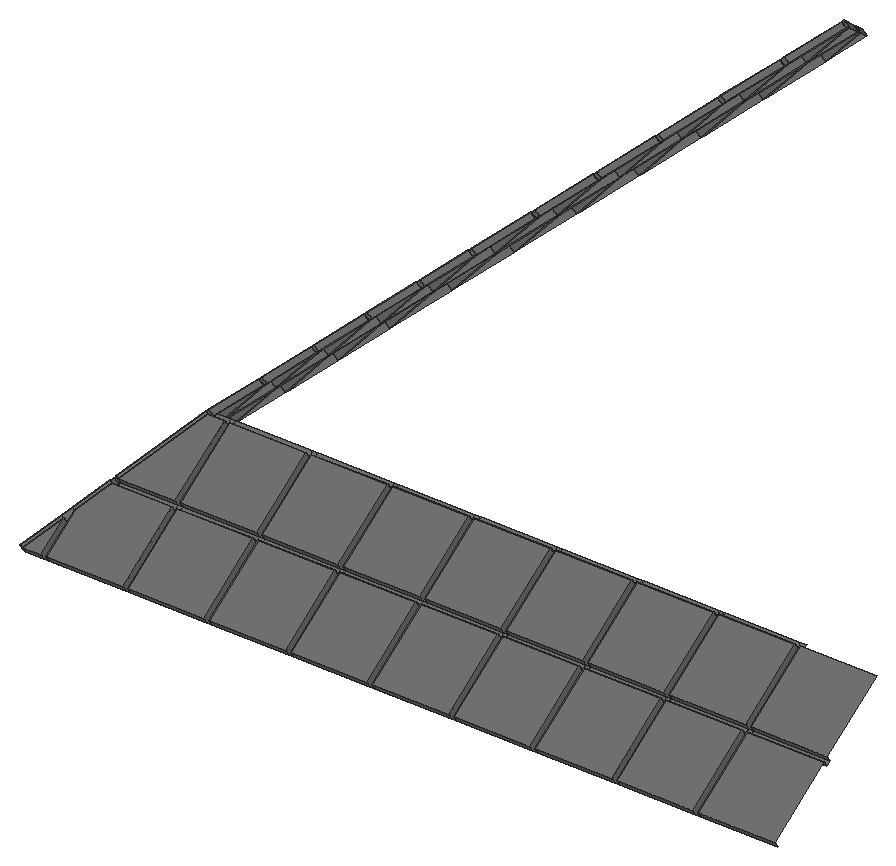
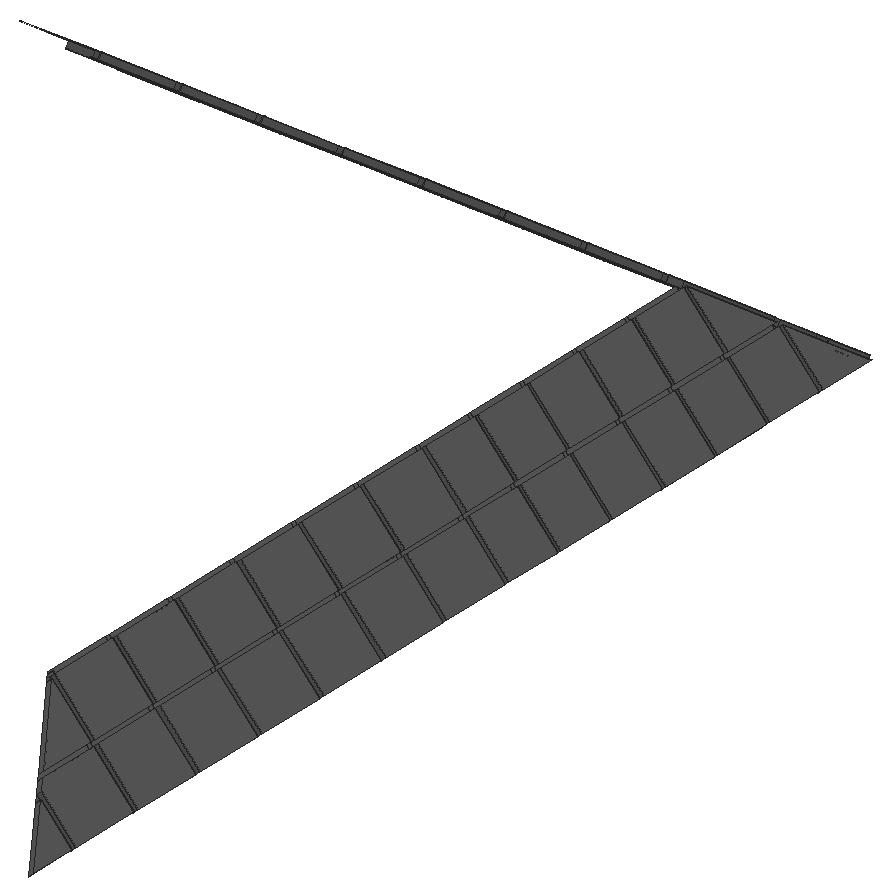
# SketchUp Ruby script. Lengths in inches.
U = 1.inch
M = Sketchup.active_model
def pt(a) = Geom::Point3d.new(a.map { |v| v * U })
def face(e, loops, mat)
  f = e.add_face(loops[0].map { |a| pt(a) })
  loops[1..].each { |l| e.add_face(l.map { |a| pt(a) }).erase! }
  f.material = f.back_material = mat if mat
  f
end
# faces: each face lists its corners as indices into pts; further lists are holes
def faces(e, pts, list, mat = nil) = list.each { |f| face(e, (f[0].is_a?(Array) ? f : [f]).map { |l| l.map { |i| pts[i] } }, mat) }
# xy, xz, yz: faces in a plane at the given z, y or x. An outline is a flat list of corners, or four numbers for a rectangle; further outlines are holes
def ring(l) = l.size == 4 ? [[l[0], l[1]], [l[2], l[1]], [l[2], l[3]], [l[0], l[3]]] : l.each_slice(2).to_a
def flat(e, list, mat, &to3) = list.each { |f| face(e, (f[0].is_a?(Array) ? f : [f]).map { |l| ring(l).map { |u, v| to3.(u, v) } }, mat) }
def xy(e, z, list, mat = nil) = flat(e, list, mat) { |x, y| [x, y, z] }
def xz(e, y, list, mat = nil) = flat(e, list, mat) { |x, z| [x, y, z] }
def yz(e, x, list, mat = nil) = flat(e, list, mat) { |y, z| [x, y, z] }
def lines(e, pts, list) = list.each { |a, b| e.add_line(pt(pts[a]), pt(pts[b])) }
# prism: a flat outline (further loops are holes) pulled along v
def prism(e, loops, v, mat = nil)
  f = face(e, loops, mat); d = Geom::Vector3d.new(v.map { |x| x * U })
  f.pushpull(f.normal.samedirection?(d) ? d.length : -d.length)
end
def box(e, o, s, mat = nil) = prism(e, [[o, [o[0] + s[0], o[1], o[2]], [o[0] + s[0], o[1] + s[1], o[2]], [o[0], o[1] + s[1], o[2]]]], [0, 0, s[2]], mat)
def at(x, y, z, deg = 0) = Geom::Transformation.translation(pt([x, y, z])) * Geom::Transformation.rotation(ORIGIN, Z_AXIS, deg.degrees)
def axes(o, x, y, z) = Geom::Transformation.new([*x, 0, *y, 0, *z, 0, *pt(o).to_a, 1])
def part(name) = M.definitions.add(name)
# library, detail: a bought-in or finely detailed component or shape, given as its bounding box
def library(name, o, s) = part(name).tap { |d| box(d.entities, o, s) }
def detail(e, o, s) = box(e.add_group.entities, o, s)
def put(e, d, t, mat = nil) = e.add_instance(d, t).tap { |i| i.material = mat if mat }
def group(e, t, mat = nil) = e.add_group.tap { |g| g.transformation = t; g.material = mat if mat }.entities
root = M.entities
M.materials.add("[Color M05]").color = [114, 114, 114]
xz(root,317.375,[[346.61,416.3,345.12,417.63,357.02,430.92,358.51,429.58]],"[Color M05]")
xz(root,318.58,[[346.61,416.3,358.51,429.58,357.02,430.92,345.12,417.63]],"[Color M05]")
xz(root,336.74,[[346.61,416.3,345.12,417.63,357.02,430.92,358.51,429.58],[359.3,430.47,357.8125,431.8,369.71,445.09,371.2,443.75]],"[Color M05]")
xz(root,337.95,[[346.61,416.3,358.51,429.58,357.02,430.92,345.12,417.63],[359.3,430.47,371.2,443.75,369.71,445.09,357.8125,431.8]],"[Color M05]")
xz(root,356.11,[[346.61,416.3,345.12,417.63,357.02,430.92,358.51,429.58],[359.3,430.47,357.8125,431.8,369.71,445.09,371.2,443.75]],"[Color M05]")
xz(root,357.32,[[346.61,416.3,358.51,429.58,357.02,430.92,345.12,417.63],[359.3,430.47,371.2,443.75,369.71,445.09,357.8125,431.8]],"[Color M05]")
xz(root,375.48,[[346.61,416.3,345.12,417.63,357.02,430.92,358.51,429.58],[359.3,430.47,357.8125,431.8,369.71,445.09,371.2,443.75]],"[Color M05]")
xz(root,376.69,[[346.61,416.3,358.51,429.58,357.02,430.92,345.12,417.63],[359.3,430.47,371.2,443.75,369.71,445.09,357.8125,431.8]],"[Color M05]")
xz(root,394.85,[[346.61,416.3,345.12,417.63,357.02,430.92,358.51,429.58],[359.3,430.47,357.8125,431.8,369.71,445.09,371.2,443.75]],"[Color M05]")
xz(root,396.0625,[[346.61,416.3,358.51,429.58,357.02,430.92,345.12,417.63],[359.3,430.47,371.2,443.75,369.71,445.09,357.8125,431.8]],"[Color M05]")
xz(root,414.22,[[346.61,416.3,345.12,417.63,357.02,430.92,358.51,429.58],[359.3,430.47,357.8125,431.8,369.71,445.09,371.2,443.75]],"[Color M05]")
xz(root,415.43,[[346.61,416.3,358.51,429.58,357.02,430.92,345.12,417.63],[359.3,430.47,371.2,443.75,369.71,445.09,357.8125,431.8]],"[Color M05]")
xz(root,433.3,[[346.61,416.3,345.12,417.63,357.02,430.92,358.51,429.58],[359.3,430.47,357.8125,431.8,369.71,445.09,371.2,443.75]],"[Color M05]")
xz(root,434.8,[[346.61,416.3,358.51,429.58,357.02,430.92,345.12,417.63],[359.3,430.47,371.2,443.75,369.71,445.09,357.8125,431.8]],"[Color M05]")
xz(root,456.21,[[346.61,416.3,345.12,417.63,357.02,430.92,358.51,429.58],[359.3,430.47,357.8125,431.8,369.71,445.09,371.2,443.75]],"[Color M05]")
xz(root,457.71,[[346.61,416.3,358.51,429.58,357.02,430.92,345.12,417.63],[359.3,430.47,371.2,443.75,369.71,445.09,357.8125,431.8]],"[Color M05]")
xz(root,479.13,[[346.61,416.3,345.12,417.63,357.02,430.92,358.51,429.58],[359.3,430.47,357.8125,431.8,369.71,445.09,371.2,443.75]],"[Color M05]")
xz(root,480.63,[[346.61,416.3,358.51,429.58,357.02,430.92,345.12,417.63],[359.3,430.47,371.2,443.75,369.71,445.09,357.8125,431.8]],"[Color M05]")
xz(root,502.04,[[346.61,416.3,345.12,417.63,357.02,430.92,358.51,429.58],[359.3,430.47,357.8125,431.8,369.71,445.09,371.2,443.75]],"[Color M05]")
xz(root,503.54,[[346.61,416.3,358.51,429.58,357.02,430.92,345.12,417.63],[359.3,430.47,371.2,443.75,369.71,445.09,357.8125,431.8]],"[Color M05]")
xz(root,524.95,[[346.61,416.3,345.12,417.63,357.02,430.92,358.51,429.58],[359.3,430.47,357.8125,431.8,369.71,445.09,371.2,443.75]],"[Color M05]")
xz(root,526.45,[[346.61,416.3,358.51,429.58,357.02,430.92,345.12,417.63],[359.3,430.47,371.2,443.75,369.71,445.09,357.8125,431.8]],"[Color M05]")
xz(root,547.87,[[346.61,416.3,345.12,417.63,357.02,430.92,358.51,429.58],[359.3,430.47,357.8125,431.8,369.71,445.09,371.2,443.75]],"[Color M05]")
xz(root,549.37,[[346.61,416.3,358.51,429.58,357.02,430.92,345.12,417.63],[359.3,430.47,371.2,443.75,369.71,445.09,357.8125,431.8]],"[Color M05]")
xz(root,570.78,[[346.61,416.3,345.12,417.63,357.02,430.92,358.51,429.58],[359.3,430.47,357.8125,431.8,369.71,445.09,371.2,443.75],[371.2,443.75,371.73,444.35,370.24,445.68,369.71,445.09]],"[Color M05]")
xz(root,572.28,[[346.61,416.3,358.51,429.58,357.02,430.92,345.12,417.63],[359.3,430.47,370.75,443.25,369.26,444.59,357.8125,431.8]],"[Color M05]")
xz(root,593.69,[[346.61,416.3,345.12,417.63,355.23,428.92,356.72,427.59]],"[Color M05]")
xz(root,595.19,[[346.61,416.3,355.74,426.49,354.25,427.82,345.12,417.63]],"[Color M05]")
yz(root,352.12,[[299.21,416.3,307.625,422.45,306.44,424.0625,298.03,417.91]],"[Color M05]")
yz(root,353.62,[[299.21,416.3,298.03,417.91,308.73,425.74,309.91,424.125]],"[Color M05]")
yz(root,376.12,[[299.21,416.3,317.375,429.58,316.19,431.2,298.03,417.91],[318.58,430.47,336.74,443.75,335.5625,445.37,317.4,432.08]],"[Color M05]")
yz(root,377.62,[[299.21,416.3,298.03,417.91,316.19,431.2,317.375,429.58],[318.58,430.47,317.4,432.08,335.5625,445.37,336.74,443.75]],"[Color M05]")
yz(root,400.12,[[299.21,416.3,317.375,429.58,316.19,431.2,298.03,417.91],[318.58,430.47,336.74,443.75,335.5625,445.37,317.4,432.08]],"[Color M05]")
yz(root,401.62,[[299.21,416.3,298.03,417.91,316.19,431.2,317.375,429.58],[318.58,430.47,317.4,432.08,335.5625,445.37,336.74,443.75]],"[Color M05]")
yz(root,424.12,[[299.21,416.3,317.375,429.58,316.19,431.2,298.03,417.91],[318.58,430.47,336.74,443.75,335.5625,445.37,317.4,432.08]],"[Color M05]")
yz(root,425.62,[[299.21,416.3,298.03,417.91,316.19,431.2,317.375,429.58],[318.58,430.47,317.4,432.08,335.5625,445.37,336.74,443.75]],"[Color M05]")
yz(root,448.12,[[299.21,416.3,317.375,429.58,316.19,431.2,298.03,417.91],[318.58,430.47,336.74,443.75,335.5625,445.37,317.4,432.08]],"[Color M05]")
yz(root,449.62,[[299.21,416.3,298.03,417.91,316.19,431.2,317.375,429.58],[318.58,430.47,317.4,432.08,335.5625,445.37,336.74,443.75]],"[Color M05]")
yz(root,472.12,[[299.21,416.3,317.375,429.58,316.19,431.2,298.03,417.91],[318.58,430.47,336.74,443.75,335.5625,445.37,317.4,432.08]],"[Color M05]")
yz(root,473.62,[[299.21,416.3,298.03,417.91,316.19,431.2,317.375,429.58],[318.58,430.47,317.4,432.08,335.5625,445.37,336.74,443.75]],"[Color M05]")
yz(root,496.12,[[299.21,416.3,317.375,429.58,316.19,431.2,298.03,417.91],[318.58,430.47,336.74,443.75,335.5625,445.37,317.4,432.08]],"[Color M05]")
yz(root,497.62,[[299.21,416.3,298.03,417.91,316.19,431.2,317.375,429.58],[318.58,430.47,317.4,432.08,335.5625,445.37,336.74,443.75]],"[Color M05]")
yz(root,520.12,[[299.21,416.3,317.375,429.58,316.19,431.2,298.03,417.91],[318.58,430.47,336.74,443.75,335.5625,445.37,317.4,432.08]],"[Color M05]")
yz(root,521.62,[[299.21,416.3,298.03,417.91,316.19,431.2,317.375,429.58],[318.58,430.47,317.4,432.08,335.5625,445.37,336.74,443.75]],"[Color M05]")
yz(root,544.12,[[299.21,416.3,317.375,429.58,316.19,431.2,298.03,417.91],[318.58,430.47,336.74,443.75,335.5625,445.37,317.4,432.08]],"[Color M05]")
yz(root,545.62,[[299.21,416.3,298.03,417.91,316.19,431.2,317.375,429.58],[318.58,430.47,317.4,432.08,335.5625,445.37,336.74,443.75]],"[Color M05]")
p = [[346.61,299.21,416.3],[352.12,299.21,416.3],[352.12,298.03,417.91],[346.61,298.03,417.91],[352.12,307.625,422.45],[352.12,306.44,424.0625],
  [353.62,299.21,416.3],[376.12,299.21,416.3],[376.12,298.03,417.91],[353.62,298.03,417.91],[377.62,299.21,416.3],[400.12,299.21,416.3],
  [400.12,298.03,417.91],[377.62,298.03,417.91],[401.62,299.21,416.3],[424.12,299.21,416.3],[424.12,298.03,417.91],[401.62,298.03,417.91],
  [425.62,299.21,416.3],[448.12,299.21,416.3],[448.12,298.03,417.91],[425.62,298.03,417.91],[449.62,299.21,416.3],[472.12,299.21,416.3],
  [472.12,298.03,417.91],[449.62,298.03,417.91],[473.62,299.21,416.3],[496.12,299.21,416.3],[496.12,298.03,417.91],[473.62,298.03,417.91],
  [497.62,299.21,416.3],[520.12,299.21,416.3],[520.12,298.03,417.91],[497.62,298.03,417.91],[521.62,299.21,416.3],[544.12,299.21,416.3],
  [544.12,298.03,417.91],[521.62,298.03,417.91],[545.62,299.21,416.3],[568.12,299.21,416.3],[568.12,298.03,417.91],[545.62,298.03,417.91],
  [346.61,317.375,416.3],[345.12,299.21,417.63],[345.12,317.375,417.63],[350.63,307.625,423.78],[353.62,309.91,424.125],[377.62,317.375,429.58],
  [376.12,317.375,429.58],[401.62,317.375,429.58],[400.12,317.375,429.58],[425.62,317.375,429.58],[424.12,317.375,429.58],[449.62,317.375,429.58],
  [448.12,317.375,429.58],[473.62,317.375,429.58],[472.12,317.375,429.58],[497.62,317.375,429.58],[496.12,317.375,429.58],[521.62,317.375,429.58],
  [520.12,317.375,429.58],[545.62,317.375,429.58],[544.12,317.375,429.58],[346.61,318.58,416.3],[358.51,317.375,429.58],[358.51,318.58,429.58],
  [346.61,336.74,416.3],[345.12,318.58,417.63],[345.12,336.74,417.63],[346.61,337.95,416.3],[358.51,336.74,429.58],[358.51,337.95,429.58],
  [346.61,356.11,416.3],[345.12,337.95,417.63],[345.12,356.11,417.63],[346.61,357.32,416.3],[358.51,356.11,429.58],[358.51,357.32,429.58],
  [346.61,375.48,416.3],[345.12,357.32,417.63],[345.12,375.48,417.63],[358.51,375.48,429.58],[358.51,376.69,429.58],[346.61,376.69,416.3],
  [346.61,394.85,416.3],[345.12,376.69,417.63],[345.12,394.85,417.63],[346.61,396.0625,416.3],[358.51,394.85,429.58],[358.51,396.0625,429.58],
  [346.61,414.22,416.3],[345.12,396.0625,417.63],[345.12,414.22,417.63],[346.61,415.43,416.3],[358.51,414.22,429.58],[358.51,415.43,429.58],
  [346.61,433.3,416.3],[345.12,415.43,417.63],[345.12,433.3,417.63],[346.61,434.8,416.3],[358.51,433.3,429.58],[358.51,434.8,429.58],
  [346.61,456.21,416.3],[345.12,434.8,417.63],[345.12,456.21,417.63],[346.61,457.71,416.3],[358.51,456.21,429.58],[358.51,457.71,429.58],
  [346.61,479.13,416.3],[345.12,457.71,417.63],[345.12,479.13,417.63],[346.61,480.63,416.3],[358.51,479.13,429.58],[358.51,480.63,429.58],
  [346.61,502.04,416.3],[345.12,480.63,417.63],[345.12,502.04,417.63],[346.61,503.54,416.3],[358.51,502.04,429.58],[358.51,503.54,429.58],
  [346.61,524.95,416.3],[345.12,503.54,417.63],[345.12,524.95,417.63],[346.61,526.45,416.3],[358.51,524.95,429.58],[358.51,526.45,429.58],
  [346.61,547.87,416.3],[345.12,526.45,417.63],[345.12,547.87,417.63],[346.61,549.37,416.3],[358.51,547.87,429.58],[358.51,549.37,429.58],
  [346.61,570.78,416.3],[345.12,549.37,417.63],[345.12,570.78,417.63],[346.61,572.28,416.3],[358.51,570.78,429.58],[358.51,572.28,429.58],
  [346.61,593.69,416.3],[345.12,572.28,417.63],[345.12,593.69,417.63],[346.61,595.19,416.3],[356.72,593.69,427.59],[355.74,595.19,426.49],
  [346.61,609.125,416.3],[345.12,595.19,417.63],[345.12,609.125,417.63],[354.25,595.19,427.82],[352.13,309.91,425.46],[357.02,317.375,430.92],
  [357.02,318.58,430.92],[357.02,336.74,430.92],[357.02,337.95,430.92],[357.02,356.11,430.92],[357.02,357.32,430.92],[357.02,375.48,430.92],
  [357.02,376.69,430.92],[357.02,394.85,430.92],[357.02,396.0625,430.92],[357.02,414.22,430.92],[357.02,415.43,430.92],[357.02,433.3,430.92],
  [357.02,434.8,430.92],[357.02,456.21,430.92],[357.02,457.71,430.92],[357.02,479.13,430.92],[357.02,480.63,430.92],[357.02,502.04,430.92],
  [357.02,503.54,430.92],[357.02,524.95,430.92],[357.02,526.45,430.92],[357.02,547.87,430.92],[357.02,549.37,430.92],[357.02,570.78,430.92],
  [357.02,572.28,430.92],[357.02,590.97,430.92],[355.23,593.69,428.92],[376.12,316.19,431.2],[358.51,316.19,431.2],[353.62,308.73,425.74],
  [400.12,316.19,431.2],[377.62,316.19,431.2],[424.12,316.19,431.2],[401.62,316.19,431.2],[448.12,316.19,431.2],[425.62,316.19,431.2],
  [472.12,316.19,431.2],[449.62,316.19,431.2],[496.12,316.19,431.2],[473.62,316.19,431.2],[520.12,316.19,431.2],[497.62,316.19,431.2],
  [544.12,316.19,431.2],[521.62,316.19,431.2],[568.12,316.19,431.2],[545.62,316.19,431.2],[358.51,590.97,429.58],[568.12,317.375,429.58],
  [359.3,318.58,430.47],[376.12,318.58,430.47],[377.62,318.58,430.47],[400.12,318.58,430.47],[401.62,318.58,430.47],[424.12,318.58,430.47],
  [425.62,318.58,430.47],[448.12,318.58,430.47],[449.62,318.58,430.47],[472.12,318.58,430.47],[473.62,318.58,430.47],[496.12,318.58,430.47],
  [497.62,318.58,430.47],[520.12,318.58,430.47],[521.62,318.58,430.47],[544.12,318.58,430.47],[545.62,318.58,430.47],[568.12,318.58,430.47],
  [359.3,336.74,430.47],[359.3,337.95,430.47],[359.3,356.11,430.47],[359.3,357.32,430.47],[359.3,375.48,430.47],[359.3,376.69,430.47],
  [359.3,394.85,430.47],[359.3,396.0625,430.47],[359.3,414.22,430.47],[359.3,415.43,430.47],[359.3,433.3,430.47],[359.3,434.8,430.47],
  [359.3,456.21,430.47],[359.3,457.71,430.47],[359.3,479.13,430.47],[359.3,480.63,430.47],[359.3,502.04,430.47],[359.3,503.54,430.47],
  [359.3,524.95,430.47],[359.3,526.45,430.47],[359.3,547.87,430.47],[359.3,549.37,430.47],[359.3,570.78,430.47],[359.3,572.28,430.47],
  [359.3,589.76,430.47],[371.2,336.74,443.75],[359.3,317.4,432.08],[371.2,335.5625,445.37],[376.12,317.4,432.08],[400.12,317.4,432.08],
  [377.62,317.4,432.08],[424.12,317.4,432.08],[401.62,317.4,432.08],[448.12,317.4,432.08],[425.62,317.4,432.08],[472.12,317.4,432.08],
  [449.62,317.4,432.08],[496.12,317.4,432.08],[473.62,317.4,432.08],[520.12,317.4,432.08],[497.62,317.4,432.08],[544.12,317.4,432.08],
  [521.62,317.4,432.08],[568.12,317.4,432.08],[545.62,317.4,432.08],[357.8125,318.58,431.8],[357.8125,336.74,431.8],[369.71,336.74,445.09],
  [377.62,336.74,443.75],[376.12,336.74,443.75],[401.62,336.74,443.75],[400.12,336.74,443.75],[425.62,336.74,443.75],[424.12,336.74,443.75],
  [449.62,336.74,443.75],[448.12,336.74,443.75],[473.62,336.74,443.75],[472.12,336.74,443.75],[497.62,336.74,443.75],[496.12,336.74,443.75],
  [521.62,336.74,443.75],[520.12,336.74,443.75],[545.62,336.74,443.75],[544.12,336.74,443.75],[371.2,337.95,443.75],[357.8125,337.95,431.8],
  [357.8125,356.11,431.8],[371.2,356.11,443.75],[371.2,357.32,443.75],[357.8125,357.32,431.8],[357.8125,375.48,431.8],[371.2,375.48,443.75],
  [371.2,376.69,443.75],[357.8125,376.69,431.8],[357.8125,394.85,431.8],[371.2,394.85,443.75],[371.2,396.0625,443.75],[357.8125,396.0625,431.8],
  [357.8125,414.22,431.8],[371.2,414.22,443.75],[371.2,415.43,443.75],[357.8125,415.43,431.8],[357.8125,433.3,431.8],[371.2,433.3,443.75],
  [371.2,434.8,443.75],[357.8125,434.8,431.8],[357.8125,456.21,431.8],[371.2,456.21,443.75],[371.2,457.71,443.75],[357.8125,457.71,431.8],
  [357.8125,479.13,431.8],[371.2,479.13,443.75],[371.2,480.63,443.75],[357.8125,480.63,431.8],[357.8125,502.04,431.8],[371.2,502.04,443.75],
  [371.2,503.54,443.75],[357.8125,503.54,431.8],[357.8125,524.95,431.8],[371.2,524.95,443.75],[371.2,526.45,443.75],[357.8125,526.45,431.8],
  [357.8125,547.87,431.8],[371.2,547.87,443.75],[371.2,549.37,443.75],[357.8125,549.37,431.8],[357.8125,570.78,431.8],[371.2,570.78,443.75],
  [371.2,571.6,443.75],[370.75,572.28,443.25],[357.8125,572.28,431.8],[357.8125,589.76,431.8],[369.26,572.28,444.59],[369.71,337.95,445.09],
  [369.71,356.11,445.09],[369.71,357.32,445.09],[369.71,375.48,445.09],[369.71,376.69,445.09],[369.71,394.85,445.09],[369.71,396.0625,445.09],
  [369.71,414.22,445.09],[369.71,415.43,445.09],[369.71,433.3,445.09],[369.71,434.8,445.09],[369.71,456.21,445.09],[369.71,457.71,445.09],
  [369.71,479.13,445.09],[369.71,480.63,445.09],[369.71,502.04,445.09],[369.71,503.54,445.09],[369.71,524.95,445.09],[369.71,526.45,445.09],
  [369.71,547.87,445.09],[369.71,549.37,445.09],[369.71,570.78,445.09],[376.12,335.5625,445.37],[400.12,335.5625,445.37],[377.62,335.5625,445.37],
  [424.12,335.5625,445.37],[401.62,335.5625,445.37],[448.12,335.5625,445.37],[425.62,335.5625,445.37],[472.12,335.5625,445.37],[449.62,335.5625,445.37],
  [496.12,335.5625,445.37],[473.62,335.5625,445.37],[520.12,335.5625,445.37],[497.62,335.5625,445.37],[544.12,335.5625,445.37],[521.62,335.5625,445.37],
  [568.12,335.5625,445.37],[545.62,335.5625,445.37],[371.99,337.95,444.64],[376.12,337.95,444.64],[377.62,337.95,444.64],[400.12,337.95,444.64],
  [401.62,337.95,444.64],[424.12,337.95,444.64],[425.62,337.95,444.64],[448.12,337.95,444.64],[449.62,337.95,444.64],[472.12,337.95,444.64],
  [473.62,337.95,444.64],[496.12,337.95,444.64],[497.62,337.95,444.64],[520.12,337.95,444.64],[521.62,337.95,444.64],[544.12,337.95,444.64],
  [545.62,337.95,444.64],[371.99,356.11,444.64],[371.99,357.32,444.64],[371.99,375.48,444.64],[371.99,376.69,444.64],[371.99,394.85,444.64],
  [371.99,396.0625,444.64],[371.99,414.22,444.64],[371.99,415.43,444.64],[371.99,433.3,444.64],[371.99,434.8,444.64],[371.99,456.21,444.64],
  [371.99,457.71,444.64],[371.99,479.13,444.64],[371.99,480.63,444.64],[371.99,502.04,444.64],[371.99,503.54,444.64],[371.99,524.95,444.64],
  [371.99,526.45,444.64],[371.99,547.87,444.64],[371.99,549.37,444.64],[371.99,570.39,444.64],[371.73,570.78,444.35],[369.71,571.6,445.09],
  [370.24,570.78,445.68]]
faces(root,p,[[0,1,2,3],[4,0,3,5],[6,7,8,9],[10,11,12,13],[14,15,16,17],[18,19,20,21],[22,23,24,25],[26,27,28,29],
  [30,31,32,33],[34,35,36,37],[38,39,40,41],[42,0,43,44],[0,4,45,43],[1,6,46,4],[7,10,47,48],[11,14,49,50],
  [15,18,51,52],[19,22,53,54],[23,26,55,56],[27,30,57,58],[31,34,59,60],[35,38,61,62],[63,42,64,65],[66,63,67,68],
  [69,66,70,71],[72,69,73,74],[75,72,76,77],[78,75,79,80],[81,82,83,78],[84,83,85,86],[87,84,88,89],[90,87,91,92],
  [93,90,94,95],[96,93,97,98],[99,96,100,101],[102,99,103,104],[105,102,106,107],[108,105,109,110],[111,108,112,113],[114,111,115,116],
  [117,114,118,119],[120,117,121,122],[123,120,124,125],[126,123,127,128],[129,126,130,131],[132,129,133,134],[135,132,136,137],[138,135,139,140],
  [141,138,142,143],[144,141,145,146],[143,144,146,147],[148,149,44,43,45],[68,67,150,151],[74,73,152,153],[80,79,154,155],[86,85,156,157],
  [92,91,158,159],[98,97,160,161],[162,163,104,103],[110,109,164,165],[116,115,166,167],[122,121,168,169],[128,127,170,171],[134,133,172,173],
  [140,139,174,175,176],[146,145,147],[3,2,5],[9,8,177,178,179],[13,12,180,181],[17,16,182,183],[21,20,184,185],[25,24,186,187],
  [29,28,188,189],[33,32,190,191],[37,36,192,193],[41,40,194,195],[4,46,148,45],[64,46,179,178],[46,64,149,148],[196,142,176,175],
  [48,64,178,177],[50,47,181,180],[52,49,183,182],[54,51,185,184],[56,53,187,186],[58,55,189,188],[60,57,191,190],[62,59,193,192],
  [197,61,195,194],[64,198,65],[64,48,199,198],[48,47,200,199],[47,50,201,200],[50,49,202,201],[49,52,203,202],[52,51,204,203],
  [51,54,205,204],[54,53,206,205],[53,56,207,206],[56,55,208,207],[55,58,209,208],[58,57,210,209],[57,60,211,210],[60,59,212,211],
  [59,62,213,212],[62,61,214,213],[61,197,215,214],[65,70,151,150],[70,65,198,216],[71,70,216,217],[71,76,153,152],[76,71,217,218],
  [77,76,218,219],[77,81,155,154],[81,77,219,220],[220,221,82,81],[82,88,157,156],[88,82,221,222],[89,88,222,223],[89,94,159,158],
  [94,89,223,224],[95,94,224,225],[95,100,161,160],[100,95,225,226],[101,100,226,227],[101,106,163,162],[227,228,106,101],[107,106,228,229],
  [107,112,165,164],[112,107,229,230],[113,112,230,231],[113,118,167,166],[118,113,231,232],[119,118,232,233],[119,124,169,168],[124,119,233,234],
  [125,124,234,235],[125,130,171,170],[130,125,235,236],[131,130,236,237],[131,136,173,172],[136,131,237,238],[137,136,238,239],[137,196,175,174],
  [196,137,239,240],[241,198,242,243],[198,199,244,242],[200,201,245,246],[202,203,247,248],[204,205,249,250],[206,207,251,252],[208,209,253,254],
  [210,211,255,256],[212,213,257,258],[214,215,259,260],[216,198,261,262],[198,241,263,261],[199,200,264,265],[201,202,266,267],[203,204,268,269],
  [205,206,270,271],[207,208,272,273],[209,210,274,275],[211,212,276,277],[213,214,278,279],[217,216,241,280],[218,217,281,282],[219,218,283,284],
  [220,219,285,286],[287,288,221,220],[222,221,289,290],[223,222,291,292],[224,223,293,294],[225,224,295,296],[226,225,297,298],[227,226,299,300],
  [228,227,301,302],[229,228,303,304],[230,229,305,306],[231,230,307,308],[232,231,309,310],[233,232,311,312],[234,233,313,314],[235,234,315,316],
  [236,235,317,318],[237,236,319,320],[238,237,321,322],[239,238,323,324,325],[240,239,326,327],[325,240,327,328],[261,263,262],[282,281,329,330],
  [286,285,331,332],[290,289,333,334],[294,293,335,336],[298,297,337,338],[339,340,302,301],[306,305,341,342],[310,309,343,344],[314,313,345,346],
  [318,317,347,348],[322,321,349,350],[327,326,328],[242,244,351,243],[246,245,352,353],[248,247,354,355],[250,249,356,357],[252,251,358,359],
  [254,253,360,361],[256,255,362,363],[258,257,364,365],[260,259,366,367],[265,241,243,351],[267,264,353,352],[269,266,355,354],[271,268,357,356],
  [273,270,359,358],[275,272,361,360],[277,274,363,362],[279,276,365,364],[241,368,280],[241,265,369,368],[265,264,370,369],[264,267,371,370],
  [267,266,372,371],[266,269,373,372],[269,268,374,373],[268,271,375,374],[271,270,376,375],[270,273,377,376],[273,272,378,377],[272,275,379,378],
  [275,274,380,379],[274,277,381,380],[277,276,382,381],[276,279,383,382],[279,278,384,383],[280,283,330,329],[283,280,368,385],[284,283,385,386],
  [284,287,332,331],[287,284,386,387],[387,388,288,287],[288,291,334,333],[291,288,388,389],[292,291,389,390],[292,295,336,335],[295,292,390,391],
  [296,295,391,392],[296,299,338,337],[299,296,392,393],[300,299,393,394],[300,303,340,339],[394,395,303,300],[304,303,395,396],[304,307,342,341],
  [307,304,396,397],[308,307,397,398],[308,311,344,343],[311,308,398,399],[312,311,399,400],[312,315,346,345],[315,312,400,401],[316,315,401,402],
  [316,319,348,347],[319,316,402,403],[320,319,403,404],[320,323,350,349],[323,320,404,405,406],[324,323,350,407],[406,324,407,408]],"[Color M05]")
